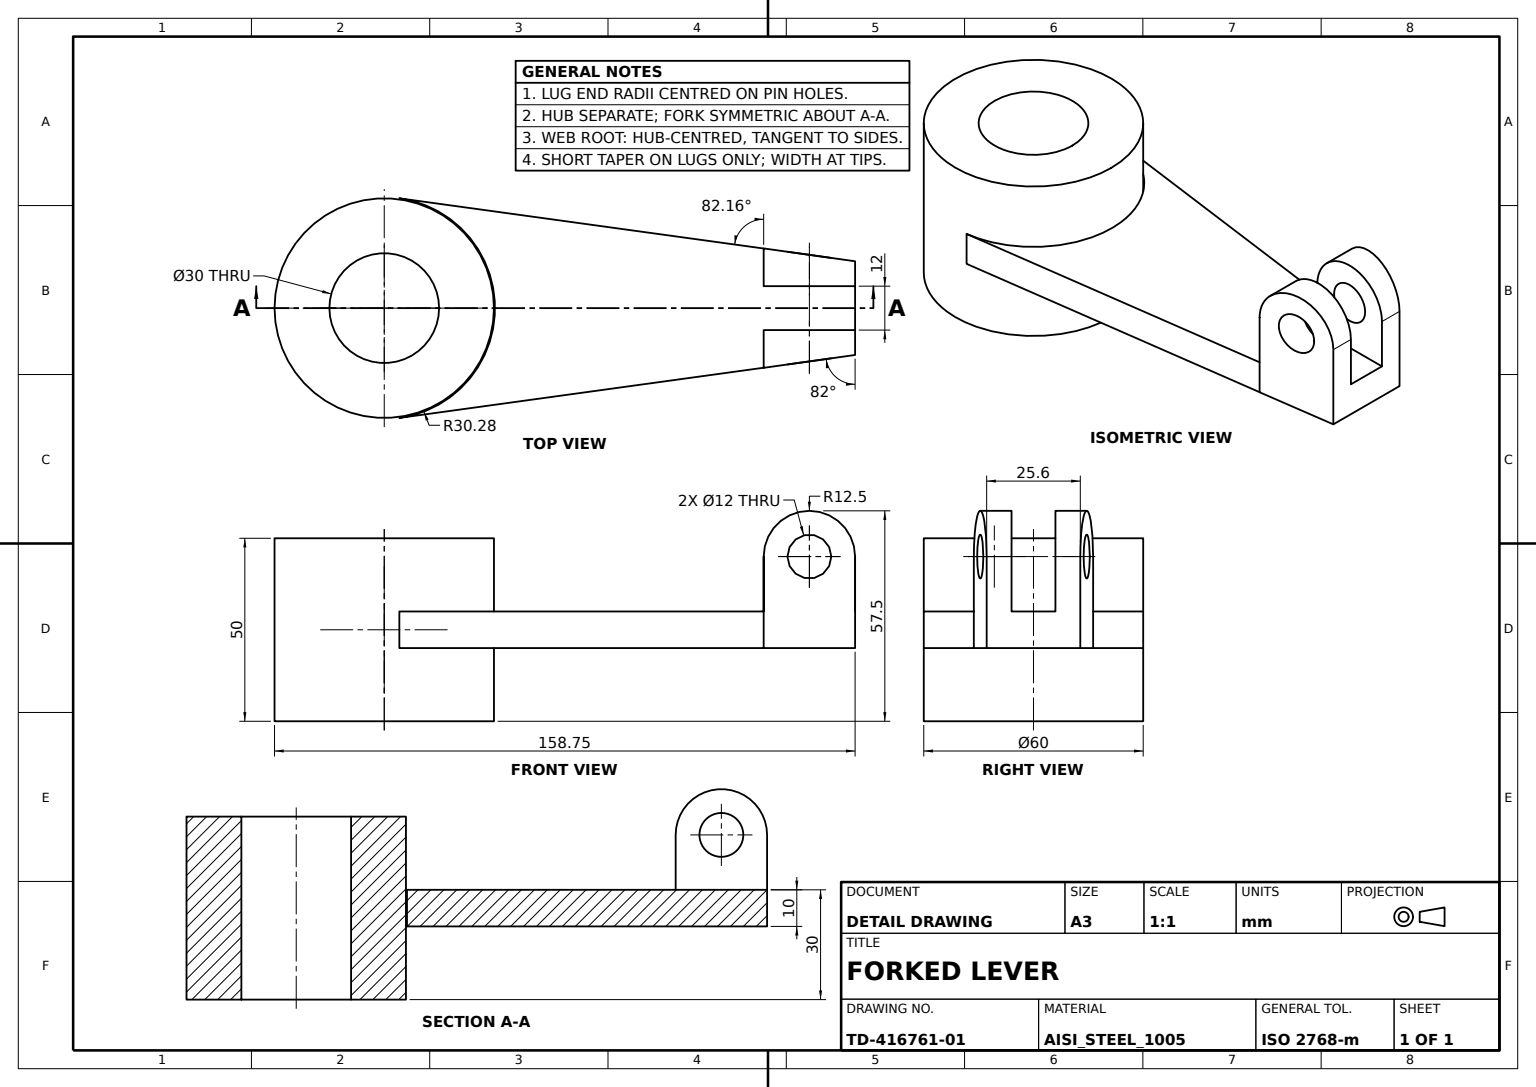
ISO-10303-21;
HEADER;
FILE_DESCRIPTION((''),'2;1');
FILE_NAME('','',(''),(''),'','','');
FILE_SCHEMA(('AUTOMOTIVE_DESIGN'));
ENDSEC;
DATA;
#1=APPLICATION_CONTEXT('');
#2=PRODUCT_CONTEXT('',#1,'mechanical');
#3=PRODUCT('','','',(#2));
#4=PRODUCT_DEFINITION_FORMATION('','',#3);
#5=PRODUCT_DEFINITION_CONTEXT('',#1,'design');
#6=PRODUCT_DEFINITION('','',#4,#5);
#7=PRODUCT_DEFINITION_SHAPE('','',#6);
#8=(LENGTH_UNIT()NAMED_UNIT(*)SI_UNIT(.MILLI.,.METRE.));
#9=(NAMED_UNIT(*)PLANE_ANGLE_UNIT()SI_UNIT($,.RADIAN.));
#10=(NAMED_UNIT(*)SI_UNIT($,.STERADIAN.)SOLID_ANGLE_UNIT());
#11=UNCERTAINTY_MEASURE_WITH_UNIT(LENGTH_MEASURE(0.005),#8,'distance_accuracy_value','');
#12=(GEOMETRIC_REPRESENTATION_CONTEXT(3)GLOBAL_UNCERTAINTY_ASSIGNED_CONTEXT((#11))GLOBAL_UNIT_ASSIGNED_CONTEXT((#8,#9,#10))REPRESENTATION_CONTEXT('',''));
#13=CARTESIAN_POINT('',(15.,0.,25.));
#14=VERTEX_POINT('',#13);
#15=CARTESIAN_POINT('',(0.,0.,25.));
#16=DIRECTION('',(0.,0.,1.));
#17=DIRECTION('',(1.,0.,0.));
#18=AXIS2_PLACEMENT_3D('',#15,#16,#17);
#19=CIRCLE('',#18,15.);
#20=EDGE_CURVE('',#14,#14,#19,.T.);
#21=ORIENTED_EDGE('',*,*,#20,.F.);
#22=EDGE_LOOP('',(#21));
#23=FACE_BOUND('',#22,.T.);
#24=CARTESIAN_POINT('',(30.,0.,25.));
#25=VERTEX_POINT('',#24);
#26=CIRCLE('',#18,30.);
#27=EDGE_CURVE('',#25,#25,#26,.T.);
#28=ORIENTED_EDGE('',*,*,#27,.T.);
#29=EDGE_LOOP('',(#28));
#30=FACE_BOUND('',#29,.T.);
#31=PLANE('',#18);
#32=ADVANCED_FACE('',(#23,#30),#31,.T.);
#33=CARTESIAN_POINT('',(15.,0.,-25.));
#34=VERTEX_POINT('',#33);
#35=CARTESIAN_POINT('',(0.,0.,-25.));
#36=AXIS2_PLACEMENT_3D('',#35,#16,#17);
#37=CIRCLE('',#36,15.);
#38=EDGE_CURVE('',#34,#34,#37,.T.);
#39=ORIENTED_EDGE('',*,*,#38,.T.);
#40=EDGE_LOOP('',(#39));
#41=FACE_BOUND('',#40,.T.);
#42=CARTESIAN_POINT('',(30.,0.,-25.));
#43=VERTEX_POINT('',#42);
#44=CIRCLE('',#36,30.);
#45=EDGE_CURVE('',#43,#43,#44,.T.);
#46=ORIENTED_EDGE('',*,*,#45,.F.);
#47=EDGE_LOOP('',(#46));
#48=FACE_BOUND('',#47,.T.);
#49=PLANE('',#36);
#50=ADVANCED_FACE('',(#41,#48),#49,.F.);
#51=ORIENTED_EDGE('',*,*,#27,.F.);
#52=EDGE_LOOP('',(#51));
#53=FACE_BOUND('',#52,.T.);
#54=ORIENTED_EDGE('',*,*,#45,.T.);
#55=EDGE_LOOP('',(#54));
#56=FACE_BOUND('',#55,.T.);
#57=DIRECTION('',(0.,0.,-1.));
#58=DIRECTION('',(-1.,0.,0.));
#59=AXIS2_PLACEMENT_3D('',#15,#57,#58);
#60=CYLINDRICAL_SURFACE('',#59,30.);
#61=ADVANCED_FACE('',(#53,#56),#60,.T.);
#62=ORIENTED_EDGE('',*,*,#38,.F.);
#63=EDGE_LOOP('',(#62));
#64=FACE_BOUND('',#63,.T.);
#65=ORIENTED_EDGE('',*,*,#20,.T.);
#66=EDGE_LOOP('',(#65));
#67=FACE_BOUND('',#66,.T.);
#68=CYLINDRICAL_SURFACE('',#59,15.);
#69=ADVANCED_FACE('',(#64,#67),#68,.F.);
#70=CLOSED_SHELL('',(#32,#50,#61,#69));
#71=MANIFOLD_SOLID_BREP('',#70);
#72=CARTESIAN_POINT('',(103.75,-16.312996,20.));
#73=VERTEX_POINT('',#72);
#74=CARTESIAN_POINT('',(103.75,-6.,20.));
#75=VERTEX_POINT('',#74);
#76=CARTESIAN_POINT('',(103.75,-15.,20.));
#77=DIRECTION('',(0.,1.,0.));
#78=VECTOR('',#77,1000.);
#79=LINE('',#76,#78);
#80=EDGE_CURVE('',#73,#75,#79,.T.);
#81=ORIENTED_EDGE('',*,*,#80,.T.);
#82=CARTESIAN_POINT('',(103.75,-6.,5.));
#83=VERTEX_POINT('',#82);
#84=VECTOR('',#57,1000.);
#85=LINE('',#74,#84);
#86=EDGE_CURVE('',#75,#83,#85,.T.);
#87=ORIENTED_EDGE('',*,*,#86,.T.);
#88=CARTESIAN_POINT('',(103.75,-16.2861,5.));
#89=VERTEX_POINT('',#88);
#90=LINE('',#88,#78);
#91=EDGE_CURVE('',#83,#89,#90,.F.);
#92=ORIENTED_EDGE('',*,*,#91,.T.);
#93=CARTESIAN_POINT('',(103.75,-16.2861,-5.));
#94=VERTEX_POINT('',#93);
#95=LINE('',#88,#84);
#96=EDGE_CURVE('',#89,#94,#95,.T.);
#97=ORIENTED_EDGE('',*,*,#96,.T.);
#98=CARTESIAN_POINT('',(103.75,-16.312996,-5.));
#99=VERTEX_POINT('',#98);
#100=LINE('',#93,#78);
#101=EDGE_CURVE('',#94,#99,#100,.F.);
#102=ORIENTED_EDGE('',*,*,#101,.T.);
#103=LINE('',#72,#84);
#104=EDGE_CURVE('',#73,#99,#103,.T.);
#105=ORIENTED_EDGE('',*,*,#104,.F.);
#106=EDGE_LOOP('',(#81,#87,#92,#97,#102,#105));
#107=FACE_BOUND('',#106,.T.);
#108=AXIS2_PLACEMENT_3D('',#76,#17,#57);
#109=PLANE('',#108);
#110=ADVANCED_FACE('',(#107),#109,.F.);
#111=CARTESIAN_POINT('',(103.75,16.2861,5.));
#112=VERTEX_POINT('',#111);
#113=CARTESIAN_POINT('',(103.75,16.2861,-5.));
#114=VERTEX_POINT('',#113);
#115=LINE('',#111,#84);
#116=EDGE_CURVE('',#112,#114,#115,.T.);
#117=ORIENTED_EDGE('',*,*,#116,.F.);
#118=CARTESIAN_POINT('',(103.75,6.,5.));
#119=VERTEX_POINT('',#118);
#120=EDGE_CURVE('',#112,#119,#90,.F.);
#121=ORIENTED_EDGE('',*,*,#120,.T.);
#122=CARTESIAN_POINT('',(103.75,6.,20.));
#123=VERTEX_POINT('',#122);
#124=VECTOR('',#16,1000.);
#125=LINE('',#122,#124);
#126=EDGE_CURVE('',#119,#123,#125,.T.);
#127=ORIENTED_EDGE('',*,*,#126,.T.);
#128=CARTESIAN_POINT('',(103.75,16.312996,20.));
#129=VERTEX_POINT('',#128);
#130=EDGE_CURVE('',#123,#129,#79,.T.);
#131=ORIENTED_EDGE('',*,*,#130,.T.);
#132=CARTESIAN_POINT('',(103.75,16.312996,-5.));
#133=VERTEX_POINT('',#132);
#134=CARTESIAN_POINT('',(103.75,16.312996,5.));
#135=LINE('',#134,#84);
#136=EDGE_CURVE('',#129,#133,#135,.T.);
#137=ORIENTED_EDGE('',*,*,#136,.T.);
#138=EDGE_CURVE('',#133,#114,#100,.F.);
#139=ORIENTED_EDGE('',*,*,#138,.T.);
#140=EDGE_LOOP('',(#117,#121,#127,#131,#137,#139));
#141=FACE_BOUND('',#140,.T.);
#142=ADVANCED_FACE('',(#141),#109,.F.);
#143=CARTESIAN_POINT('',(4.129858,-30.,-5.));
#144=VERTEX_POINT('',#143);
#145=DIRECTION('',(0.990657181,0.136375767,0.));
#146=VECTOR('',#145,1000.);
#147=LINE('',#143,#146);
#148=EDGE_CURVE('',#144,#94,#147,.T.);
#149=ORIENTED_EDGE('',*,*,#148,.F.);
#150=CARTESIAN_POINT('',(4.129858,30.,-5.));
#151=VERTEX_POINT('',#150);
#152=CARTESIAN_POINT('',(0.,0.,-5.));
#153=AXIS2_PLACEMENT_3D('',#152,#57,#17);
#154=CIRCLE('',#153,30.282928);
#155=EDGE_CURVE('',#151,#144,#154,.T.);
#156=ORIENTED_EDGE('',*,*,#155,.F.);
#157=DIRECTION('',(-0.990657181,0.136375767,0.));
#158=VECTOR('',#157,1000.);
#159=LINE('',#113,#158);
#160=EDGE_CURVE('',#114,#151,#159,.T.);
#161=ORIENTED_EDGE('',*,*,#160,.F.);
#162=ORIENTED_EDGE('',*,*,#138,.F.);
#163=CARTESIAN_POINT('',(128.75,12.799476,-5.));
#164=VERTEX_POINT('',#163);
#165=CARTESIAN_POINT('',(113.092455,15.,-5.));
#166=DIRECTION('',(-0.990268069,0.139173101,0.));
#167=VECTOR('',#166,1000.);
#168=LINE('',#165,#167);
#169=EDGE_CURVE('',#133,#164,#168,.F.);
#170=ORIENTED_EDGE('',*,*,#169,.T.);
#171=CARTESIAN_POINT('',(128.75,-12.799476,-5.));
#172=VERTEX_POINT('',#171);
#173=CARTESIAN_POINT('',(128.75,-15.,-5.));
#174=LINE('',#173,#78);
#175=EDGE_CURVE('',#172,#164,#174,.T.);
#176=ORIENTED_EDGE('',*,*,#175,.F.);
#177=CARTESIAN_POINT('',(113.092455,-15.,-5.));
#178=DIRECTION('',(0.990268069,0.139173101,0.));
#179=VECTOR('',#178,1000.);
#180=LINE('',#177,#179);
#181=EDGE_CURVE('',#99,#172,#180,.T.);
#182=ORIENTED_EDGE('',*,*,#181,.F.);
#183=ORIENTED_EDGE('',*,*,#101,.F.);
#184=EDGE_LOOP('',(#149,#156,#161,#162,#170,#176,#182,#183));
#185=FACE_BOUND('',#184,.T.);
#186=AXIS2_PLACEMENT_3D('',#152,#57,#58);
#187=PLANE('',#186);
#188=ADVANCED_FACE('',(#185),#187,.T.);
#189=CARTESIAN_POINT('',(4.129858,-30.,5.));
#190=VERTEX_POINT('',#189);
#191=LINE('',#189,#146);
#192=EDGE_CURVE('',#190,#89,#191,.T.);
#193=ORIENTED_EDGE('',*,*,#192,.F.);
#194=LINE('',#189,#84);
#195=EDGE_CURVE('',#190,#144,#194,.T.);
#196=ORIENTED_EDGE('',*,*,#195,.T.);
#197=ORIENTED_EDGE('',*,*,#148,.T.);
#198=ORIENTED_EDGE('',*,*,#96,.F.);
#199=EDGE_LOOP('',(#193,#196,#197,#198));
#200=FACE_BOUND('',#199,.T.);
#201=DIRECTION('',(-0.136375767,0.990657181,0.));
#202=DIRECTION('',(-0.990657181,-0.136375767,0.));
#203=AXIS2_PLACEMENT_3D('',#189,#201,#202);
#204=PLANE('',#203);
#205=ADVANCED_FACE('',(#200),#204,.F.);
#206=CARTESIAN_POINT('',(4.129858,30.,5.));
#207=VERTEX_POINT('',#206);
#208=LINE('',#111,#158);
#209=EDGE_CURVE('',#112,#207,#208,.T.);
#210=ORIENTED_EDGE('',*,*,#209,.T.);
#211=CARTESIAN_POINT('',(0.,0.,5.));
#212=AXIS2_PLACEMENT_3D('',#211,#57,#17);
#213=CIRCLE('',#212,30.282928);
#214=EDGE_CURVE('',#207,#190,#213,.T.);
#215=ORIENTED_EDGE('',*,*,#214,.T.);
#216=ORIENTED_EDGE('',*,*,#192,.T.);
#217=ORIENTED_EDGE('',*,*,#91,.F.);
#218=CARTESIAN_POINT('',(128.75,-6.,5.));
#219=VERTEX_POINT('',#218);
#220=CARTESIAN_POINT('',(98.75,-6.,5.));
#221=VECTOR('',#17,1000.);
#222=LINE('',#220,#221);
#223=EDGE_CURVE('',#83,#219,#222,.T.);
#224=ORIENTED_EDGE('',*,*,#223,.T.);
#225=CARTESIAN_POINT('',(128.75,6.,5.));
#226=VERTEX_POINT('',#225);
#227=CARTESIAN_POINT('',(128.75,0.,5.));
#228=LINE('',#227,#78);
#229=EDGE_CURVE('',#219,#226,#228,.T.);
#230=ORIENTED_EDGE('',*,*,#229,.T.);
#231=CARTESIAN_POINT('',(98.75,6.,5.));
#232=LINE('',#231,#221);
#233=EDGE_CURVE('',#119,#226,#232,.T.);
#234=ORIENTED_EDGE('',*,*,#233,.F.);
#235=ORIENTED_EDGE('',*,*,#120,.F.);
#236=EDGE_LOOP('',(#210,#215,#216,#217,#224,#230,#234,#235));
#237=FACE_BOUND('',#236,.T.);
#238=AXIS2_PLACEMENT_3D('',#211,#57,#58);
#239=PLANE('',#238);
#240=ADVANCED_FACE('',(#237),#239,.F.);
#241=CARTESIAN_POINT('',(110.25,15.399481,20.));
#242=VERTEX_POINT('',#241);
#243=CARTESIAN_POINT('',(116.25,14.556236,20.));
#244=DIRECTION('',(0.139173101,0.990268069,0.));
#245=AXIS2_PLACEMENT_3D('',#243,#244,#166);
#246=ELLIPSE('',#245,6.058965,6.);
#247=EDGE_CURVE('',#242,#242,#246,.F.);
#248=ORIENTED_EDGE('',*,*,#247,.T.);
#249=EDGE_LOOP('',(#248));
#250=FACE_BOUND('',#249,.T.);
#251=CARTESIAN_POINT('',(128.75,12.799476,20.));
#252=VERTEX_POINT('',#251);
#253=ELLIPSE('',#245,12.622845,12.5);
#254=EDGE_CURVE('',#252,#129,#253,.F.);
#255=ORIENTED_EDGE('',*,*,#254,.F.);
#256=LINE('',#163,#84);
#257=EDGE_CURVE('',#164,#252,#256,.F.);
#258=ORIENTED_EDGE('',*,*,#257,.F.);
#259=ORIENTED_EDGE('',*,*,#169,.F.);
#260=ORIENTED_EDGE('',*,*,#136,.F.);
#261=EDGE_LOOP('',(#255,#258,#259,#260));
#262=FACE_BOUND('',#261,.T.);
#263=CARTESIAN_POINT('',(113.092455,15.,0.));
#264=AXIS2_PLACEMENT_3D('',#263,#244,#166);
#265=PLANE('',#264);
#266=ADVANCED_FACE('',(#250,#262),#265,.T.);
#267=CARTESIAN_POINT('',(128.75,-6.,20.));
#268=VERTEX_POINT('',#267);
#269=CARTESIAN_POINT('',(116.25,-6.,20.));
#270=DIRECTION('',(0.,-1.,0.));
#271=AXIS2_PLACEMENT_3D('',#269,#270,#57);
#272=CIRCLE('',#271,12.5);
#273=EDGE_CURVE('',#268,#75,#272,.T.);
#274=ORIENTED_EDGE('',*,*,#273,.T.);
#275=ORIENTED_EDGE('',*,*,#80,.F.);
#276=CARTESIAN_POINT('',(128.75,-12.799476,20.));
#277=VERTEX_POINT('',#276);
#278=CARTESIAN_POINT('',(116.25,-14.556236,20.));
#279=DIRECTION('',(0.139173101,-0.990268069,0.));
#280=AXIS2_PLACEMENT_3D('',#278,#279,#178);
#281=ELLIPSE('',#280,12.622845,12.5);
#282=EDGE_CURVE('',#277,#73,#281,.T.);
#283=ORIENTED_EDGE('',*,*,#282,.F.);
#284=CARTESIAN_POINT('',(128.75,-15.,20.));
#285=LINE('',#284,#78);
#286=EDGE_CURVE('',#277,#268,#285,.T.);
#287=ORIENTED_EDGE('',*,*,#286,.T.);
#288=EDGE_LOOP('',(#274,#275,#283,#287));
#289=FACE_BOUND('',#288,.T.);
#290=CARTESIAN_POINT('',(116.25,-15.,20.));
#291=AXIS2_PLACEMENT_3D('',#290,#77,#16);
#292=CYLINDRICAL_SURFACE('',#291,12.5);
#293=ADVANCED_FACE('',(#289),#292,.T.);
#294=CARTESIAN_POINT('',(128.75,6.,20.));
#295=VERTEX_POINT('',#294);
#296=LINE('',#225,#124);
#297=EDGE_CURVE('',#226,#295,#296,.T.);
#298=ORIENTED_EDGE('',*,*,#297,.F.);
#299=ORIENTED_EDGE('',*,*,#229,.F.);
#300=CARTESIAN_POINT('',(128.75,-6.,32.5));
#301=LINE('',#300,#84);
#302=EDGE_CURVE('',#268,#219,#301,.T.);
#303=ORIENTED_EDGE('',*,*,#302,.F.);
#304=ORIENTED_EDGE('',*,*,#286,.F.);
#305=LINE('',#171,#124);
#306=EDGE_CURVE('',#172,#277,#305,.T.);
#307=ORIENTED_EDGE('',*,*,#306,.F.);
#308=ORIENTED_EDGE('',*,*,#175,.T.);
#309=ORIENTED_EDGE('',*,*,#257,.T.);
#310=EDGE_CURVE('',#295,#252,#285,.T.);
#311=ORIENTED_EDGE('',*,*,#310,.F.);
#312=EDGE_LOOP('',(#298,#299,#303,#304,#307,#308,#309,#311));
#313=FACE_BOUND('',#312,.T.);
#314=AXIS2_PLACEMENT_3D('',#173,#58,#16);
#315=PLANE('',#314);
#316=ADVANCED_FACE('',(#313),#315,.F.);
#317=ORIENTED_EDGE('',*,*,#209,.F.);
#318=ORIENTED_EDGE('',*,*,#116,.T.);
#319=ORIENTED_EDGE('',*,*,#160,.T.);
#320=LINE('',#206,#84);
#321=EDGE_CURVE('',#207,#151,#320,.T.);
#322=ORIENTED_EDGE('',*,*,#321,.F.);
#323=EDGE_LOOP('',(#317,#318,#319,#322));
#324=FACE_BOUND('',#323,.T.);
#325=DIRECTION('',(-0.136375767,-0.990657181,0.));
#326=DIRECTION('',(0.990657181,-0.136375767,0.));
#327=AXIS2_PLACEMENT_3D('',#111,#325,#326);
#328=PLANE('',#327);
#329=ADVANCED_FACE('',(#324),#328,.F.);
#330=CARTESIAN_POINT('',(116.25,6.,20.));
#331=AXIS2_PLACEMENT_3D('',#330,#77,#16);
#332=CIRCLE('',#331,12.5);
#333=EDGE_CURVE('',#123,#295,#332,.T.);
#334=ORIENTED_EDGE('',*,*,#333,.T.);
#335=ORIENTED_EDGE('',*,*,#310,.T.);
#336=ORIENTED_EDGE('',*,*,#254,.T.);
#337=ORIENTED_EDGE('',*,*,#130,.F.);
#338=EDGE_LOOP('',(#334,#335,#336,#337));
#339=FACE_BOUND('',#338,.T.);
#340=ADVANCED_FACE('',(#339),#292,.T.);
#341=CARTESIAN_POINT('',(116.25,6.,26.));
#342=VERTEX_POINT('',#341);
#343=CIRCLE('',#331,6.);
#344=EDGE_CURVE('',#342,#342,#343,.T.);
#345=ORIENTED_EDGE('',*,*,#344,.F.);
#346=EDGE_LOOP('',(#345));
#347=FACE_BOUND('',#346,.T.);
#348=ORIENTED_EDGE('',*,*,#247,.F.);
#349=EDGE_LOOP('',(#348));
#350=FACE_BOUND('',#349,.T.);
#351=CYLINDRICAL_SURFACE('',#291,6.);
#352=ADVANCED_FACE('',(#347,#350),#351,.F.);
#353=ORIENTED_EDGE('',*,*,#321,.T.);
#354=ORIENTED_EDGE('',*,*,#155,.T.);
#355=ORIENTED_EDGE('',*,*,#195,.F.);
#356=ORIENTED_EDGE('',*,*,#214,.F.);
#357=EDGE_LOOP('',(#353,#354,#355,#356));
#358=FACE_BOUND('',#357,.T.);
#359=CYLINDRICAL_SURFACE('',#238,30.282928);
#360=ADVANCED_FACE('',(#358),#359,.F.);
#361=CARTESIAN_POINT('',(122.25,-13.712991,20.));
#362=VERTEX_POINT('',#361);
#363=ELLIPSE('',#280,6.058965,6.);
#364=EDGE_CURVE('',#362,#362,#363,.T.);
#365=ORIENTED_EDGE('',*,*,#364,.T.);
#366=EDGE_LOOP('',(#365));
#367=FACE_BOUND('',#366,.T.);
#368=CARTESIAN_POINT('',(116.25,-6.,14.));
#369=VERTEX_POINT('',#368);
#370=CIRCLE('',#271,6.);
#371=EDGE_CURVE('',#369,#369,#370,.T.);
#372=ORIENTED_EDGE('',*,*,#371,.F.);
#373=EDGE_LOOP('',(#372));
#374=FACE_BOUND('',#373,.T.);
#375=ADVANCED_FACE('',(#367,#374),#351,.F.);
#376=ORIENTED_EDGE('',*,*,#371,.T.);
#377=EDGE_LOOP('',(#376));
#378=FACE_BOUND('',#377,.T.);
#379=ORIENTED_EDGE('',*,*,#223,.F.);
#380=ORIENTED_EDGE('',*,*,#86,.F.);
#381=ORIENTED_EDGE('',*,*,#273,.F.);
#382=ORIENTED_EDGE('',*,*,#302,.T.);
#383=EDGE_LOOP('',(#379,#380,#381,#382));
#384=FACE_BOUND('',#383,.T.);
#385=CARTESIAN_POINT('',(98.75,-6.,32.5));
#386=AXIS2_PLACEMENT_3D('',#385,#270,#57);
#387=PLANE('',#386);
#388=ADVANCED_FACE('',(#378,#384),#387,.F.);
#389=ORIENTED_EDGE('',*,*,#344,.T.);
#390=EDGE_LOOP('',(#389));
#391=FACE_BOUND('',#390,.T.);
#392=ORIENTED_EDGE('',*,*,#233,.T.);
#393=ORIENTED_EDGE('',*,*,#297,.T.);
#394=ORIENTED_EDGE('',*,*,#333,.F.);
#395=ORIENTED_EDGE('',*,*,#126,.F.);
#396=EDGE_LOOP('',(#392,#393,#394,#395));
#397=FACE_BOUND('',#396,.T.);
#398=AXIS2_PLACEMENT_3D('',#231,#77,#16);
#399=PLANE('',#398);
#400=ADVANCED_FACE('',(#391,#397),#399,.F.);
#401=ORIENTED_EDGE('',*,*,#181,.T.);
#402=ORIENTED_EDGE('',*,*,#306,.T.);
#403=ORIENTED_EDGE('',*,*,#282,.T.);
#404=ORIENTED_EDGE('',*,*,#104,.T.);
#405=EDGE_LOOP('',(#401,#402,#403,#404));
#406=FACE_BOUND('',#405,.T.);
#407=ORIENTED_EDGE('',*,*,#364,.F.);
#408=EDGE_LOOP('',(#407));
#409=FACE_BOUND('',#408,.T.);
#410=CARTESIAN_POINT('',(113.092455,-15.,0.));
#411=AXIS2_PLACEMENT_3D('',#410,#279,#178);
#412=PLANE('',#411);
#413=ADVANCED_FACE('',(#406,#409),#412,.T.);
#414=CLOSED_SHELL('',(#110,#142,#188,#205,#240,#266,#293,#316,#329,#340,#352,#360,#375,#388,#400,#413));
#415=MANIFOLD_SOLID_BREP('',#414);
#416=ADVANCED_BREP_SHAPE_REPRESENTATION('',(#71,#415),#12);
#417=SHAPE_DEFINITION_REPRESENTATION(#7,#416);
ENDSEC;
END-ISO-10303-21;
